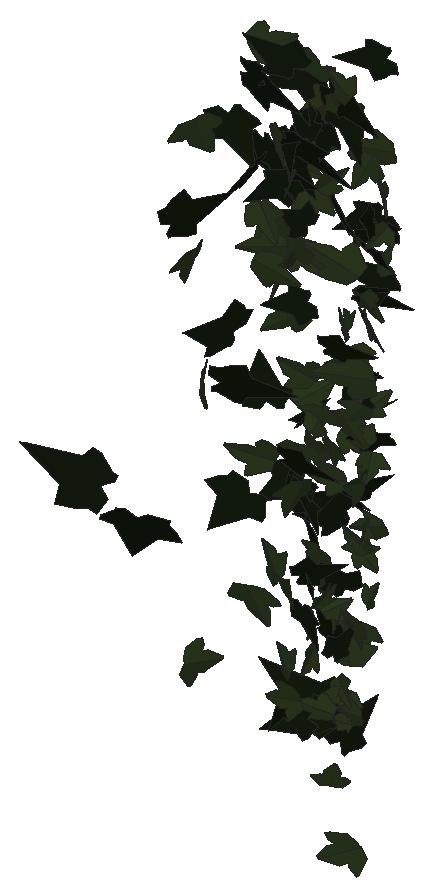
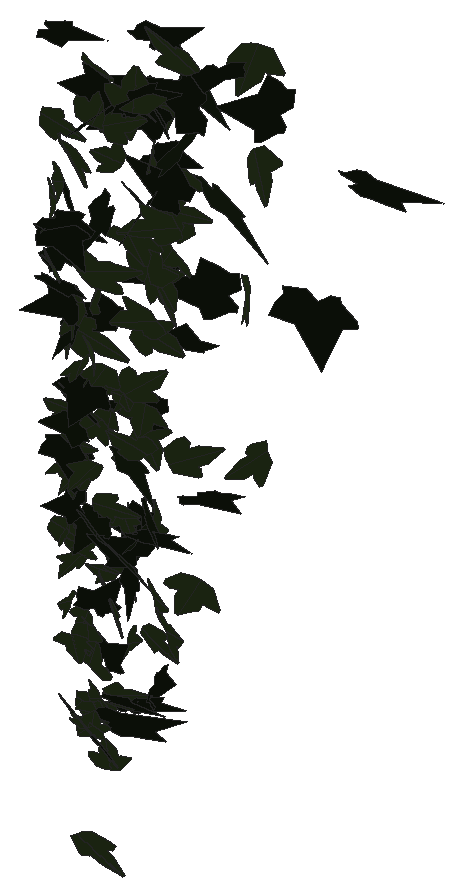
# SketchUp Ruby script. Lengths in inches.
U = 1.inch
M = Sketchup.active_model
def pt(a) = Geom::Point3d.new(a.map { |v| v * U })
def face(e, loops, mat)
  f = e.add_face(loops[0].map { |a| pt(a) })
  loops[1..].each { |l| e.add_face(l.map { |a| pt(a) }).erase! }
  f.material = f.back_material = mat if mat
  f
end
# faces: each face lists its corners as indices into pts; further lists are holes
def faces(e, pts, list, mat = nil) = list.each { |f| face(e, (f[0].is_a?(Array) ? f : [f]).map { |l| l.map { |i| pts[i] } }, mat) }
# xy, xz, yz: faces in a plane at the given z, y or x. An outline is a flat list of corners, or four numbers for a rectangle; further outlines are holes
def ring(l) = l.size == 4 ? [[l[0], l[1]], [l[2], l[1]], [l[2], l[3]], [l[0], l[3]]] : l.each_slice(2).to_a
def flat(e, list, mat, &to3) = list.each { |f| face(e, (f[0].is_a?(Array) ? f : [f]).map { |l| ring(l).map { |u, v| to3.(u, v) } }, mat) }
def xy(e, z, list, mat = nil) = flat(e, list, mat) { |x, y| [x, y, z] }
def xz(e, y, list, mat = nil) = flat(e, list, mat) { |x, z| [x, y, z] }
def yz(e, x, list, mat = nil) = flat(e, list, mat) { |y, z| [x, y, z] }
def lines(e, pts, list) = list.each { |a, b| e.add_line(pt(pts[a]), pt(pts[b])) }
# prism: a flat outline (further loops are holes) pulled along v
def prism(e, loops, v, mat = nil)
  f = face(e, loops, mat); d = Geom::Vector3d.new(v.map { |x| x * U })
  f.pushpull(f.normal.samedirection?(d) ? d.length : -d.length)
end
def box(e, o, s, mat = nil) = prism(e, [[o, [o[0] + s[0], o[1], o[2]], [o[0] + s[0], o[1] + s[1], o[2]], [o[0], o[1] + s[1], o[2]]]], [0, 0, s[2]], mat)
def at(x, y, z, deg = 0) = Geom::Transformation.translation(pt([x, y, z])) * Geom::Transformation.rotation(ORIGIN, Z_AXIS, deg.degrees)
def axes(o, x, y, z) = Geom::Transformation.new([*x, 0, *y, 0, *z, 0, *pt(o).to_a, 1])
def part(name) = M.definitions.add(name)
# library, detail: a bought-in or finely detailed component or shape, given as its bounding box
def library(name, o, s) = part(name).tap { |d| box(d.entities, o, s) }
def detail(e, o, s) = box(e.add_group.entities, o, s)
def put(e, d, t, mat = nil) = e.add_instance(d, t).tap { |i| i.material = mat if mat }
def group(e, t, mat = nil) = e.add_group.tap { |g| g.transformation = t; g.material = mat if mat }.entities
root = M.entities
M.materials.add("1026 AP 7946 SUNNY SIDE UP").color = [254, 231, 186]
M.materials.add("efeu1").color = [18, 25, 13]
M.materials.add("efeu2").color = [43, 57, 29]
c1 = part("ivyleaf_10")
p = [[0,0.5,-0.03],[-0.0625,2.02,-0.43],[-0.19,2.01,-0.46],[-0.54,1.05,-0.29],[-0.52,0.625,-0.18],[-0.83,0.76,-0.28],
  [-1.16,0.64,-0.33],[-1.15,0.33,-0.24],[-0.77,-0.39,0.02],[-0.3,-0.51,0.16],[0.04,-0.48,0.23],[-0.02,2.01,-0.4375],
  [-0.06,2.01,-0.43],[0.04,-0.49,0.23],[0.67,-0.49,0.14],[1.38,0.36,-0.2],[1.375,0.51,-0.24],[0.81,0.65,-0.19],
  [0.62,0.59,-0.15],[0.6,1.09,-0.28],[0.5,1.23,-0.31]]
faces(c1.entities,p,[[0,1,2,3,4,5,6,7,8,9,10],[11,12,0,13,14,15,16,17,18,19,20]],"efeu2")
c2 = part("ivyleaf_9")
p = [[1.54,2.16,1.25],[1.36,2.04,1.19],[-0.21,0.99,0.68],[-0.71,1.11,0.82],[-0.85,0.86,0.67],[-0.8,0.17,0.21],
  [-0.9,-0.01,0.1],[-0.67,-0.16,-0.02],[-0.08,-0.08,-0.05],[-0.03,-0.6,-0.4],[0.65,-0.88,-0.66],[0.83,-0.6,-0.49],
  [1.29,-0.42,-0.43],[1.8125,-0.07,-0.26],[1.21,0.44,0.15]]
faces(c2.entities,p,[[0,1,2,3,4,5,6,7,8,9,10,11,12,13,14]],"efeu1")
put(root,c1,axes([135.0625,209.38,255.31],[0.25036,-0.06231,0.31306],[-0.40947,0.15948,0.17498],[-0.26605,-0.3041,0.02528]),"1026 AP 7946 SUNNY SIDE UP")
put(root,c1,axes([134.62,210,264.51],[0.14656,0.08738,0.33573],[0.37684,0.2201,-0.13032],[-0.37236,0.25714,0.00025]),"1026 AP 7946 SUNNY SIDE UP")
put(root,c1,axes([134.96,206.89,266.74],[-0.29368,-0.30873,-0.1681],[0.16045,0.12664,-0.37042],[0.52378,-0.2119,0.01922]),"1026 AP 7946 SUNNY SIDE UP")
put(root,c2,axes([134.57,209.16,266.77],[0.26093,-0.03824,-0.36864],[0.5638,0.04839,0.16636],[0.04422,-0.39127,0.05426]),"1026 AP 7946 SUNNY SIDE UP")
put(root,c2,axes([135.23,208.21,257.7],[-0.416,-0.20861,0.07837],[-0.06433,-0.07238,-0.34606],[0.34382,-0.26594,0.03008]),"1026 AP 7946 SUNNY SIDE UP")
put(root,c1,axes([135.51,208.47,258.51],[-0.12392,-0.08912,-0.32639],[-0.42026,-0.17189,0.11748],[-0.30067,0.27699,-0.02969]),"1026 AP 7946 SUNNY SIDE UP")
put(root,c1,axes([135.29,206.375,264.11],[-0.00312,-0.39726,-0.0433],[0.00049,0.03978,-0.40903],[0.62778,-0.002,0.0001]),"1026 AP 7946 SUNNY SIDE UP")
put(root,c2,axes([135.44,209.7,257.45],[-0.42114,-0.10478,0.10085],[-0.12632,-0.06365,-0.29521],[0.18754,-0.27818,0.02761]),"1026 AP 7946 SUNNY SIDE UP")
put(root,c1,axes([134.875,209.13,267.56],[0.36701,-0.1126,-0.27343],[0.41616,-0.0497,0.26184],[-0.17745,-0.34945,0.04856]),"1026 AP 7946 SUNNY SIDE UP")
put(root,c1,axes([134.93,210.12,262.43],[0.24528,0.04823,0.2976],[0.43991,0.07121,-0.16763],[-0.13476,0.32024,-0.00554]),"1026 AP 7946 SUNNY SIDE UP")
put(root,c1,axes([135.41,209.25,262.78],[-0.08948,-0.31579,0.11326],[-0.02459,-0.11071,-0.33118],[0.52613,-0.05888,0.00378]),"1026 AP 7946 SUNNY SIDE UP")
put(root,c2,axes([135.28,209.74,257.95],[-0.23921,0.0552,-0.27673],[0.36242,-0.14137,-0.16504],[-0.23454,-0.27474,0.02722]),"1026 AP 7946 SUNNY SIDE UP")
put(root,c2,axes([135.25,209.77,264.67],[0.24185,-0.20136,-0.20897],[-0.2049,0.15415,-0.26001],[0.39856,0.20144,-0.00687]),"1026 AP 7946 SUNNY SIDE UP")
put(root,c1,axes([135.1,209.18,263.4375],[0.40708,-0.09067,0.2347],[0.31722,-0.11085,-0.28164],[0.22047,0.32692,-0.02812]),"1026 AP 7946 SUNNY SIDE UP")
put(root,c2,axes([135.2,207.6875,266.69],[-0.02078,-0.29677,-0.19103],[0.02619,0.18313,-0.30487],[0.54822,-0.02,0.00732]),"1026 AP 7946 SUNNY SIDE UP")
put(root,c1,axes([135.39,209.125,262.44],[0.22584,-0.31227,0.04506],[0.01412,-0.04594,-0.35419],[0.49601,0.14349,-0.01043]),"1026 AP 7946 SUNNY SIDE UP")
put(root,c1,axes([135.63,206.3,261.09],[-0.01752,0.04353,0.40966],[-0.40382,0.3039,-0.03994],[-0.48175,-0.25632,0.01858]),"1026 AP 7946 SUNNY SIDE UP")
put(root,c2,axes([135.17,205.94,264.98],[0.0643,0.08439,0.43025],[0.50027,0.27231,-0.08729],[-0.44454,0.31866,-0.036]),"1026 AP 7946 SUNNY SIDE UP")
put(root,c2,axes([135.12,208.93,265.49],[0.26848,-0.34383,0.00061],[-0.02111,-0.0095,-0.39518],[0.54024,0.1705,-0.01575]),"1026 AP 7946 SUNNY SIDE UP")
put(root,c2,axes([135.55,209.86,266.88],[0.01461,-0.17273,-0.30728],[0.03528,-0.29646,0.17644],[-0.53948,-0.02407,0.00322]),"1026 AP 7946 SUNNY SIDE UP")
put(root,c1,axes([135.67,209.26,261.55],[-0.20749,-0.13874,0.26814],[-0.24331,-0.2112,-0.19743],[0.39612,-0.2024,0.01918]),"1026 AP 7946 SUNNY SIDE UP")
put(root,c2,axes([135,209.22,264.68],[0.15068,-0.06357,0.3553],[0.36719,-0.25567,-0.11677],[0.41215,0.25102,-0.02587]),"1026 AP 7946 SUNNY SIDE UP")
put(root,c2,axes([135.71,209.79,259.07],[-0.17312,0.28317,0.01795],[-0.03458,0.0084,-0.31243],[-0.44461,-0.11091,0.01731]),"1026 AP 7946 SUNNY SIDE UP")
put(root,c1,axes([135.56,209.83,266.8],[-0.38978,-0.23143,-0.06158],[-0.09276,-0.02227,0.34839],[-0.36369,0.25372,-0.02286]),"1026 AP 7946 SUNNY SIDE UP")
put(root,c1,axes([135.48,209.94,263.98],[0.52053,0.01383,-0.04367],[-0.0644,-0.03264,-0.34006],[-0.028,0.33215,-0.02963]),"1026 AP 7946 SUNNY SIDE UP")
put(root,c1,axes([135.55,209.36,262.91],[-0.51799,0.03335,0.02204],[0.03794,0.02868,0.33978],[0.04922,0.32886,-0.02991]),"1026 AP 7946 SUNNY SIDE UP")
put(root,c1,axes([135.49,208.03,255.58],[-0.5059,0.00101,-0.0995],[0.15093,-0.03414,-0.32996],[-0.01695,-0.33418,0.03143]),"1026 AP 7946 SUNNY SIDE UP")
put(root,c2,axes([135.88,208.82,267.59],[-0.01922,0.07093,0.29604],[-0.46476,0.0005,-0.0131],[-0.00556,-0.28722,0.0713]),"1026 AP 7946 SUNNY SIDE UP")
put(root,c1,axes([135.93,208.29,263.65],[-0.05031,-0.01557,0.3045],[-0.29964,-0.22652,-0.03486],[0.3563,-0.19269,0.01368]),"1026 AP 7946 SUNNY SIDE UP")
put(root,c1,axes([135.42,209.77,259.31],[0.28915,0.06974,-0.24327],[0.3212,0.12221,0.20144],[0.21722,-0.27355,0.02596]),"1026 AP 7946 SUNNY SIDE UP")
put(root,c2,axes([135.75,209.62,256.47],[0.24676,-0.07186,-0.23806],[-0.35337,0.05758,-0.17565],[0.13948,0.27299,-0.02383]),"1026 AP 7946 SUNNY SIDE UP")
put(root,c1,axes([136,209.26,260.22],[-0.21798,-0.11858,-0.25313],[-0.33424,-0.12463,0.18529],[-0.2674,0.25244,-0.02526]),"1026 AP 7946 SUNNY SIDE UP")
put(root,c2,axes([135.93,208.62,265.02],[-0.01831,-0.02726,-0.296],[0.01495,-0.28729,0.02602],[-0.45334,-0.00838,0.01281]),"1026 AP 7946 SUNNY SIDE UP")
put(root,c2,axes([135.59,209.63,257.27],[0.09386,-0.28271,0.1097],[0.03178,-0.1062,-0.29828],[0.47485,0.06299,-0.00172]),"1026 AP 7946 SUNNY SIDE UP")
put(root,c1,axes([135.9,209.96,266.24],[-0.01996,-0.02539,0.35064],[0.00186,-0.34075,-0.02812],[0.53691,0.00024,0.01313]),"1026 AP 7946 SUNNY SIDE UP")
put(root,c1,axes([135.7,208.51,266.09],[-0.14266,0.13911,-0.25642],[0.17268,-0.2249,-0.1715],[-0.41495,-0.14142,0.01679]),"1026 AP 7946 SUNNY SIDE UP")
put(root,c2,axes([136.47,201.79,261.18],[-0.46768,-0.18103,-0.27795],[-0.40021,-0.09531,0.35574],[-0.31539,0.38939,-0.03924]),"1026 AP 7946 SUNNY SIDE UP")
put(root,c1,axes([135.99,208.625,265.06],[-0.00136,-0.0774,-0.28264],[-0.03658,0.27302,-0.0778],[0.44607,0.02216,-0.00724]),"1026 AP 7946 SUNNY SIDE UP")
put(root,c2,axes([135.71,209.6,256.88],[-0.06193,0.01499,0.31079],[0.4401,0.11597,0.03239],[-0.17821,0.28118,-0.028]),"1026 AP 7946 SUNNY SIDE UP")
put(root,c1,axes([135.69,208.1,264.49],[0.38178,0.00016,0.20371],[0.30814,-0.04202,-0.2481],[0.04153,0.31031,-0.03185]),"1026 AP 7946 SUNNY SIDE UP")
put(root,c2,axes([136.17,207.29,265.99],[-0.3263,0.2419,-0.17936],[0.15039,-0.14863,-0.32848],[-0.44518,-0.22751,0.02049]),"1026 AP 7946 SUNNY SIDE UP")
put(root,c2,axes([136.28,208.81,264.04],[-0.17538,0.17952,0.17512],[-0.16858,0.13168,-0.21626],[-0.34907,-0.15379,0.01646]),"1026 AP 7946 SUNNY SIDE UP")
put(root,c2,axes([136.14,207.69,260.45],[-0.45997,-0.04205,0.1017],[0.14716,0.04163,0.30348],[-0.08322,0.30599,-0.02545]),"1026 AP 7946 SUNNY SIDE UP")
put(root,c2,axes([135.89,208.73,266.05],[-0.18779,-0.03085,-0.26948],[0.40711,-0.0655,-0.11428],[-0.07459,-0.27983,0.05471]),"1026 AP 7946 SUNNY SIDE UP")
put(root,c2,axes([136.14,203.54,259.48],[0.41306,0.22547,-0.22487],[-0.22735,-0.16756,-0.35646],[-0.43953,0.29856,-0.02695]),"1026 AP 7946 SUNNY SIDE UP")
put(root,c1,axes([136.37,209.7,257.78],[0.03209,-0.03032,-0.26337],[-0.40375,0.01351,-0.02271],[0.02512,0.25593,-0.02848]),"1026 AP 7946 SUNNY SIDE UP")
put(root,c2,axes([136.27,209.02,266.33],[-0.40476,0.08845,-0.06445],[0.07627,-0.05153,-0.27875],[-0.15283,-0.25997,0.03157]),"1026 AP 7946 SUNNY SIDE UP")
put(root,c2,axes([136.53,206.09,262.86],[-0.36624,0.37652,0.10776],[-0.12588,0.07068,-0.45464],[-0.60052,-0.24444,0.02958]),"1026 AP 7946 SUNNY SIDE UP")
put(root,c2,axes([136.6,209.11,252.74],[-0.5442,-0.22189,-0.15734],[-0.21974,-0.06228,0.42258],[-0.36079,0.37262,-0.02005]),"1026 AP 7946 SUNNY SIDE UP")
put(root,c1,axes([135.83,208.01,263.32],[-0.1217,-0.02685,-0.3075],[0.45196,-0.0934,-0.06871],[-0.13259,-0.29372,0.04805]),"1026 AP 7946 SUNNY SIDE UP")
put(root,c1,axes([136.29,209.48,255.5],[0.1297,-0.1961,-0.15286],[-0.10851,0.13054,-0.21813],[0.37004,0.10701,-0.01038]),"1026 AP 7946 SUNNY SIDE UP")
put(root,c2,axes([136.63,209.61,257.2],[-0.41692,0.32223,0.09781],[-0.12454,0.05518,-0.42877],[-0.51249,-0.27555,0.02462]),"1026 AP 7946 SUNNY SIDE UP")
put(root,c2,axes([136.375,208.67,262.34],[-0.01837,-0.16326,-0.21241],[-0.02884,-0.20445,0.1674],[-0.41138,0.02162,-0.00225]),"1026 AP 7946 SUNNY SIDE UP")
put(root,c1,axes([136.41,210,261.14],[0.12204,-0.01479,0.27664],[-0.29719,0.19596,0.06852],[-0.30103,-0.19945,0.04451]),"1026 AP 7946 SUNNY SIDE UP")
put(root,c1,axes([136.61,209.75,262.72],[0.22391,0.12346,0.33234],[-0.45479,-0.14677,0.18894],[0.29504,-0.31993,0.03903]),"1026 AP 7946 SUNNY SIDE UP")
put(root,c2,axes([135.86,206.6875,261.17],[0.3207,0.05129,0.31556],[0.48632,-0.0042,-0.21166],[-0.03918,0.36773,-0.04424]),"1026 AP 7946 SUNNY SIDE UP")
put(root,c2,axes([136.25,208.25,253.3],[-0.01208,-0.03194,-0.29715],[0.28002,-0.22811,0.01981],[-0.35993,-0.17639,0.02539]),"1026 AP 7946 SUNNY SIDE UP")
put(root,c2,axes([136.51,209.43,254.3],[0.09559,-0.07011,0.23978],[-0.18782,0.20081,0.09547],[-0.33358,-0.13316,0.01496]),"1026 AP 7946 SUNNY SIDE UP")
put(root,c2,axes([136.56,208.4375,252.84],[-0.29958,-0.08728,0.17055],[-0.21128,-0.10165,-0.21447],[0.20583,-0.23138,0.02808]),"1026 AP 7946 SUNNY SIDE UP")
put(root,c1,axes([136.48,209.82,266.17],[-0.2791,-0.22212,-0.16969],[-0.17921,-0.11792,0.2919],[-0.39487,0.21052,-0.01254]),"1026 AP 7946 SUNNY SIDE UP")
put(root,c2,axes([136.29,209.71,264.1875],[0.42033,-0.1603,-0.21132],[-0.28787,0.09144,-0.32029],[0.28944,0.32373,-0.01166]),"1026 AP 7946 SUNNY SIDE UP")
put(root,c2,axes([136.25,209.42,266.11],[-0.03778,-0.27164,0.18962],[0.00238,-0.18619,-0.28161],[0.51731,-0.01898,0.01514]),"1026 AP 7946 SUNNY SIDE UP")
put(root,c1,axes([136.29,208.97,265.8],[-0.03475,-0.07175,-0.27462],[0.23528,0.22114,-0.07292],[0.36405,-0.14977,0.02091]),"1026 AP 7946 SUNNY SIDE UP")
put(root,c1,axes([136.21,209.16,258.61],[-0.23957,0.06201,0.24943],[0.37553,-0.04607,0.16696],[0.11402,0.28203,-0.0258]),"1026 AP 7946 SUNNY SIDE UP")
put(root,c2,axes([136.08,208.58,266.01],[0.62132,-0.03225,0.07893],[0.11479,-0.04517,-0.40677],[0.06306,0.39999,-0.03718]),"1026 AP 7946 SUNNY SIDE UP")
put(root,c1,axes([136.51,208.32,259.15],[-0.41207,-0.03408,-0.00894],[0.01853,-0.02517,-0.27103],[0.05203,-0.26099,0.02573]),"1026 AP 7946 SUNNY SIDE UP")
put(root,c2,axes([136.45,209.8,257.49],[0.38726,0.03148,-0.10996],[-0.17419,0.04063,-0.25033],[-0.01927,0.2654,0.05297]),"1026 AP 7946 SUNNY SIDE UP")
put(root,c1,axes([136.76,209.53,266.95],[0.18763,0.02401,0.24885],[-0.36715,0.08443,0.11074],[-0.1036,-0.25572,0.05825]),"1026 AP 7946 SUNNY SIDE UP")
put(root,c1,axes([136.46,209.625,260.5625],[-0.19784,-0.19374,-0.16184],[0.17313,0.11337,-0.23589],[0.3507,-0.16526,0.02515]),"1026 AP 7946 SUNNY SIDE UP")
put(root,c1,axes([136.42,210.01,258.69],[0.11134,0.21207,0.17279],[0.06873,0.16086,-0.22925],[-0.41836,0.08287,0.00832]),"1026 AP 7946 SUNNY SIDE UP")
put(root,c2,axes([136.66,209.57,255.43],[0.14128,0.05804,0.23275],[-0.3475,-0.05519,0.10498],[0.11578,-0.23647,0.03108]),"1026 AP 7946 SUNNY SIDE UP")
put(root,c1,axes([136.7,208.78,259.86],[-0.32886,-0.08894,0.07498],[-0.09093,-0.05035,-0.23327],[0.15675,-0.21582,0.02198]),"1026 AP 7946 SUNNY SIDE UP")
put(root,c2,axes([136.4,209.97,266.23],[0.06901,-0.35974,0.00929],[-0.00398,-0.01145,-0.3734],[0.56592,0.04379,-0.00376]),"1026 AP 7946 SUNNY SIDE UP")
put(root,c2,axes([136.54,209.9,260.32],[0.3522,0.14862,-0.04421],[-0.03971,-0.04087,-0.27641],[-0.24036,0.22453,-0.01912]),"1026 AP 7946 SUNNY SIDE UP")
put(root,c1,axes([136.54,209.12,264.89],[-0.03663,-0.16112,0.21564],[0.03189,0.20934,0.16882],[-0.41526,0.03029,-0.00605]),"1026 AP 7946 SUNNY SIDE UP")
put(root,c1,axes([136.59,208.64,254.27],[0.02869,0.12123,-0.2472],[-0.03934,-0.23939,-0.1276],[-0.42187,0.03057,-0.00491]),"1026 AP 7946 SUNNY SIDE UP")
put(root,c2,axes([136.93,208.7,252.9],[-0.27365,0.03784,0.17197],[-0.26762,-0.0159,-0.1794],[-0.02536,-0.24048,0.03748]),"1026 AP 7946 SUNNY SIDE UP")
put(root,c1,axes([136.71,208.04,258.45],[-0.09767,-0.33805,0.07785],[-0.01016,-0.07758,-0.35446],[0.54524,-0.062,0.00734]),"1026 AP 7946 SUNNY SIDE UP")
put(root,c1,axes([136.88,208.68,253.03],[0.07119,0.07736,0.23785],[-0.2816,-0.14787,0.08652],[0.25843,-0.18244,0.02876]),"1026 AP 7946 SUNNY SIDE UP")
put(root,c2,axes([136.24,209.74,266.73],[0.05555,-0.06391,-0.36671],[0.55261,0.08896,0.02002],[0.13179,-0.3461,0.07063]),"1026 AP 7946 SUNNY SIDE UP")
put(root,c1,axes([136.9,207.47,254.57],[0.16278,-0.04058,0.28354],[-0.36197,0.15285,0.11321],[-0.24629,-0.25146,0.02101]),"1026 AP 7946 SUNNY SIDE UP")
put(root,c1,axes([136.62,208.64,259.54],[0.10153,0.12142,-0.2074],[0.10411,0.19167,0.14161],[0.35568,-0.09076,0.01776]),"1026 AP 7946 SUNNY SIDE UP")
put(root,c1,axes([136.95,207.54,253.82],[0.16216,-0.0973,-0.25937],[-0.33787,0.13255,-0.14299],[0.25552,0.23702,-0.02446]),"1026 AP 7946 SUNNY SIDE UP")
put(root,c1,axes([136.89,208.47,256.81],[-0.31218,0.02974,0.1217],[-0.18841,-0.00879,-0.20553],[-0.03305,-0.23077,0.02214]),"1026 AP 7946 SUNNY SIDE UP")
put(root,c2,axes([136.42,208.06,258.99],[0.2955,-0.04594,0.21087],[0.29751,-0.08236,-0.19823],[0.14338,0.26559,-0.02325]),"1026 AP 7946 SUNNY SIDE UP")
put(root,c1,axes([136.65,209.58,259.39],[-0.33492,0.03531,-0.15823],[0.22212,-0.07249,-0.21911],[-0.11059,-0.25252,0.03914]),"1026 AP 7946 SUNNY SIDE UP")
put(root,c1,axes([137.04,209.79,258.89],[0.1824,0.03511,0.22283],[-0.34424,0.01757,0.11823],[0.00145,-0.24463,0.039]),"1026 AP 7946 SUNNY SIDE UP")
put(root,c1,axes([136.77,207.63,256.12],[-0.3138,0.17333,0.11593],[0.14828,-0.06128,0.27155],[0.28819,0.22026,-0.01349]),"1026 AP 7946 SUNNY SIDE UP")
put(root,c1,axes([136.76,209.91,260.78],[0.04303,0.26777,-0.00249],[0.00239,-0.00411,-0.27731],[-0.42108,0.02734,-0.00183]),"1026 AP 7946 SUNNY SIDE UP")
put(root,c1,axes([136.92,209.51,254.8],[-0.32506,0.0546,0.06145],[-0.0982,-0.00511,-0.21932],[-0.08021,-0.21501,0.01947]),"1026 AP 7946 SUNNY SIDE UP")
put(root,c1,axes([136.84,209.33,253.13],[0.30834,0.09458,-0.06437],[-0.07624,-0.04406,-0.22379],[-0.16164,0.20121,-0.01725]),"1026 AP 7946 SUNNY SIDE UP")
put(root,c2,axes([137.05,210.22,263.92],[0.00288,-0.01817,-0.28069],[-0.15741,-0.25344,0.01525],[-0.39931,0.09977,-0.00804]),"1026 AP 7946 SUNNY SIDE UP")
put(root,c1,axes([136.98,208.13,255.375],[0.08227,-0.13235,-0.21129],[-0.12751,0.18761,-0.14546],[0.36096,0.09643,-0.00323]),"1026 AP 7946 SUNNY SIDE UP")
put(root,c1,axes([136.95,209.39,254.06],[0.54709,-0.06303,0.15934],[-0.22428,0.07537,0.3618],[-0.13763,-0.37338,0.0438]),"1026 AP 7946 SUNNY SIDE UP")
put(root,c2,axes([137.02,210.1875,263.71],[0.15862,0.13041,-0.22304],[-0.19218,-0.17978,-0.1707],[-0.349,0.15827,-0.00737]),"1026 AP 7946 SUNNY SIDE UP")
put(root,c1,axes([136.95,209.99,261.52],[-0.25665,0.18679,0.10895],[-0.1265,0.06851,-0.25472],[-0.31203,-0.18141,0.01365]),"1026 AP 7946 SUNNY SIDE UP")
put(root,c2,axes([136.8125,209.75,259.67],[-0.2335,0.18585,0.10448],[0.12248,-0.06585,0.24397],[0.3087,0.1667,-0.01777]),"1026 AP 7946 SUNNY SIDE UP")
put(root,c1,axes([136.93,208.85,259.13],[-0.3082,0.11495,0.02587],[-0.04779,-0.00362,-0.23334],[-0.17851,-0.19749,0.01779]),"1026 AP 7946 SUNNY SIDE UP")
put(root,c1,axes([137.01,209.18,261.66],[-0.19617,0.19649,-0.04676],[-0.02645,0.04436,0.23985],[0.3164,0.12554,-0.00894]),"1026 AP 7946 SUNNY SIDE UP")
put(root,c1,axes([136.72,209.35,253.32],[0.19881,-0.02807,0.20395],[0.2859,-0.08176,-0.13195],[0.13141,0.22036,-0.02149]),"1026 AP 7946 SUNNY SIDE UP")
put(root,c1,axes([136.95,209.32,252.63],[0.31515,0.09024,0.01627],[-0.03505,0.01247,0.22553],[0.13958,-0.20062,0.01991]),"1026 AP 7946 SUNNY SIDE UP")
put(root,c1,axes([137.17,209.53,256.54],[-0.26432,0.0015,-0.15726],[-0.23726,0.03288,0.1717],[0.0365,0.22468,-0.02273]),"1026 AP 7946 SUNNY SIDE UP")
put(root,c1,axes([137,209.95,265.35],[0.44949,-0.23381,-0.02987],[-0.05707,-0.00076,-0.37969],[0.36578,0.2872,-0.02253]),"1026 AP 7946 SUNNY SIDE UP")
put(root,c2,axes([136.89,209.96,261.57],[0.30392,-0.12626,-0.12864],[-0.18266,0.0483,-0.23663],[0.21014,0.22459,-0.01964]),"1026 AP 7946 SUNNY SIDE UP")
put(root,c2,axes([137.05,209.91,258.93],[0.1863,0.19401,-0.11557],[-0.08089,-0.10124,-0.23464],[-0.34387,0.12892,-0.00742]),"1026 AP 7946 SUNNY SIDE UP")
put(root,c2,axes([136.93,208.94,254.28],[-0.19057,0.20944,0.06672],[0.06177,-0.05067,0.24884],[0.33857,0.12713,-0.00785]),"1026 AP 7946 SUNNY SIDE UP")
put(root,c1,axes([137.02,209.72,257.875],[-0.04989,-0.1064,-0.31602],[-0.1036,-0.29907,0.11237],[-0.499,0.07273,0.00826]),"1026 AP 7946 SUNNY SIDE UP")
put(root,c2,axes([136.85,208.16,256.21],[-0.0009,-0.03694,0.25951],[0.04644,-0.25042,-0.03919],[0.39795,0.02914,0.00516]),"1026 AP 7946 SUNNY SIDE UP")
put(root,c2,axes([136.91,209.8125,259.38],[-0.0408,0.20518,-0.15228],[-0.02261,0.14833,0.2139],[0.39807,0.02946,-0.00346]),"1026 AP 7946 SUNNY SIDE UP")
put(root,c1,axes([136.8125,209.98,262.11],[-0.23776,0.09035,-0.21208],[0.25956,-0.12472,-0.18157],[-0.24107,-0.22339,0.01367]),"1026 AP 7946 SUNNY SIDE UP")
put(root,c1,axes([137.02,209.75,258.26],[-0.00229,0.12003,0.22197],[-0.06722,0.21139,-0.12077],[-0.381,-0.03802,0.01997]),"1026 AP 7946 SUNNY SIDE UP")
put(root,c2,axes([136.89,209.82,257.63],[0.07215,0.06547,0.24833],[0.26405,0.17284,-0.08041],[-0.28999,0.17366,-0.01143]),"1026 AP 7946 SUNNY SIDE UP")
put(root,c2,axes([136.8125,208.04,256.44],[0.08591,0.03605,0.26291],[0.37,0.09896,-0.06577],[-0.16459,0.24128,-0.01063]),"1026 AP 7946 SUNNY SIDE UP")
put(root,c1,axes([137.01,208.38,255.7],[-0.02383,-0.2041,0.11194],[0.01648,0.10934,0.21147],[-0.36406,0.01831,0.00224]),"1026 AP 7946 SUNNY SIDE UP")
put(root,c2,axes([136.94,209.16,252.2],[-0.26721,0.31639,0.17647],[0.1508,-0.14069,0.36878],[0.54386,0.19446,-0.01555]),"1026 AP 7946 SUNNY SIDE UP")
put(root,c1,axes([136.9375,210.3,264.84],[-0.13103,0.14559,-0.23373],[0.14179,-0.20966,-0.17332],[-0.40063,-0.12182,0.01511]),"1026 AP 7946 SUNNY SIDE UP")
put(root,c2,axes([136.9,207.95,255.71],[0.11087,-0.25467,0.04779],[0.01067,-0.04774,-0.27244],[0.40731,0.07057,-0.00587]),"1026 AP 7946 SUNNY SIDE UP")
put(root,c1,axes([137.09,208.62,251.49],[-0.2966,-0.12389,0.01347],[0.00361,0.02153,0.23198],[-0.19597,0.1879,-0.01611]),"1026 AP 7946 SUNNY SIDE UP")
put(root,c1,axes([137.33,208.96,249.86],[0.36099,-0.07787,-0.24288],[-0.36215,0.05155,-0.24875],[0.14407,0.32469,-0.0167]),"1026 AP 7946 SUNNY SIDE UP")
put(root,c1,axes([136.98,204.19,256.18],[-0.02423,-0.09828,-0.39305],[0.23493,0.35124,-0.09752],[0.57231,-0.14834,0.02339]),"1026 AP 7946 SUNNY SIDE UP")
put(root,c1,axes([137.57,209.03,260.83],[-0.16252,0.06001,0.39606],[-0.5941,-0.10913,-0.08781],[0.144,-0.38251,0.08471]),"1026 AP 7946 SUNNY SIDE UP")
put(root,c2,axes([136.84,210,262.08],[0.31495,0.06896,0.1688],[0.25572,0.02714,-0.21694],[-0.11148,0.2571,-0.02075]),"1026 AP 7946 SUNNY SIDE UP")
put(root,c1,axes([137.11,209.65,254.59],[0.34952,0.03281,-0.02836],[-0.05129,0.03388,-0.22795],[-0.04394,0.22143,0.04043]),"1026 AP 7946 SUNNY SIDE UP")
put(root,c2,axes([137.09,210.21,262.57],[-0.30602,-0.10352,-0.12231],[0.18065,0.03447,-0.22589],[0.16844,-0.22505,0.02004]),"1026 AP 7946 SUNNY SIDE UP")
put(root,c1,axes([137.38,209.78,257.01],[-0.13576,-0.01632,0.21706],[-0.30437,-0.08547,-0.089],[0.1337,-0.21114,0.0178]),"1026 AP 7946 SUNNY SIDE UP")
put(root,c2,axes([136.81,208.94,261.3125],[0.17735,-0.00423,0.22293],[0.33165,-0.05274,-0.11461],[0.07655,0.23828,-0.01994]),"1026 AP 7946 SUNNY SIDE UP")
put(root,c2,axes([137.39,209.96,267.79],[-0.08819,-0.11138,-0.24112],[-0.17728,-0.20443,0.12721],[-0.36601,0.12586,-0.00351]),"1026 AP 7946 SUNNY SIDE UP")
put(root,c1,axes([137.38,209.09,252.93],[-0.03549,0.01634,0.20838],[-0.31877,0.0051,-0.02371],[-0.01084,-0.20338,0.01495]),"1026 AP 7946 SUNNY SIDE UP")
put(root,c1,axes([137.14,209.86,258.47],[0.18021,0.20092,-0.08955],[-0.05537,-0.08122,-0.23858],[-0.34046,0.11955,-0.00859]),"1026 AP 7946 SUNNY SIDE UP")
put(root,c1,axes([137.07,209.625,256.34],[0.09503,0.1825,0.13039],[0.05781,0.12005,-0.19733],[-0.34346,0.0707,0.00286]),"1026 AP 7946 SUNNY SIDE UP")
put(root,c1,axes([136.98,209.3,252.6],[0.27474,0.02344,0.12863],[0.19827,-0.00799,-0.18047],[-0.02263,0.21453,-0.0195]),"1026 AP 7946 SUNNY SIDE UP")
put(root,c1,axes([137.32,209.27,259.95],[-0.24811,-0.10675,0.11289],[-0.12887,-0.07496,-0.19617],[0.20392,-0.17725,0.01337]),"1026 AP 7946 SUNNY SIDE UP")
put(root,c2,axes([136.99,210.1,263.02],[0.3744,-0.11682,-0.07089],[0.11251,-0.00829,0.27212],[-0.18047,-0.24753,0.02257]),"1026 AP 7946 SUNNY SIDE UP")
put(root,c2,axes([137.39,209.57,264.19],[-0.01139,-0.01106,-0.25267],[-0.36912,0.07196,0.00422],[0.11272,0.23452,-0.01171]),"1026 AP 7946 SUNNY SIDE UP")
put(root,c1,axes([137.26,210.14,263.67],[0.11348,0.12367,-0.20304],[-0.14475,-0.17514,-0.14844],[-0.33704,0.11686,-0.00461]),"1026 AP 7946 SUNNY SIDE UP")
put(root,c1,axes([137.19,209.74,256.98],[0.03611,0.14918,-0.18605],[-0.04804,-0.17887,-0.15653],[-0.36622,0.03817,0.00219]),"1026 AP 7946 SUNNY SIDE UP")
put(root,c1,axes([137.54,209.85,265.75],[-0.09596,0.02085,0.27523],[-0.41151,-0.06298,-0.05692],[0.08971,-0.26659,0.03332]),"1026 AP 7946 SUNNY SIDE UP")
put(root,c1,axes([137.09,210.31,264.42],[-0.09711,0.10547,-0.25329],[0.11745,-0.23613,-0.12476],[-0.40484,-0.09381,0.02456]),"1026 AP 7946 SUNNY SIDE UP")
put(root,c1,axes([137.14,210.2,262.76],[0.27095,-0.17599,0.00034],[0.02356,0.01652,0.2528],[-0.27574,-0.17153,0.02193]),"1026 AP 7946 SUNNY SIDE UP")
put(root,c1,axes([137.08,209.84,259.66],[0.15553,0.08877,-0.21323],[0.20968,0.15977,0.13684],[0.28628,-0.16525,0.01562]),"1026 AP 7946 SUNNY SIDE UP")
put(root,c1,axes([137.21,209.21,254.88],[-0.29315,0.12206,-0.03923],[0.03498,-0.03658,-0.22902],[-0.19831,-0.18688,0.0176]),"1026 AP 7946 SUNNY SIDE UP")
put(root,c1,axes([137.09,208.52,255.54],[0.14889,0.04325,-0.19818],[0.22737,0.13024,0.10412],[0.21133,-0.1706,0.0276]),"1026 AP 7946 SUNNY SIDE UP")
put(root,c1,axes([137.18,208.7,255.44],[0.19599,-0.12957,0.10429],[0.09856,-0.08099,-0.18543],[0.2398,0.13919,-0.00902]),"1026 AP 7946 SUNNY SIDE UP")
put(root,c1,axes([137.25,209.6,255.34],[0.03107,0.07151,-0.21349],[0.04763,0.2056,0.07711],[0.34201,-0.03513,0.00865]),"1026 AP 7946 SUNNY SIDE UP")
